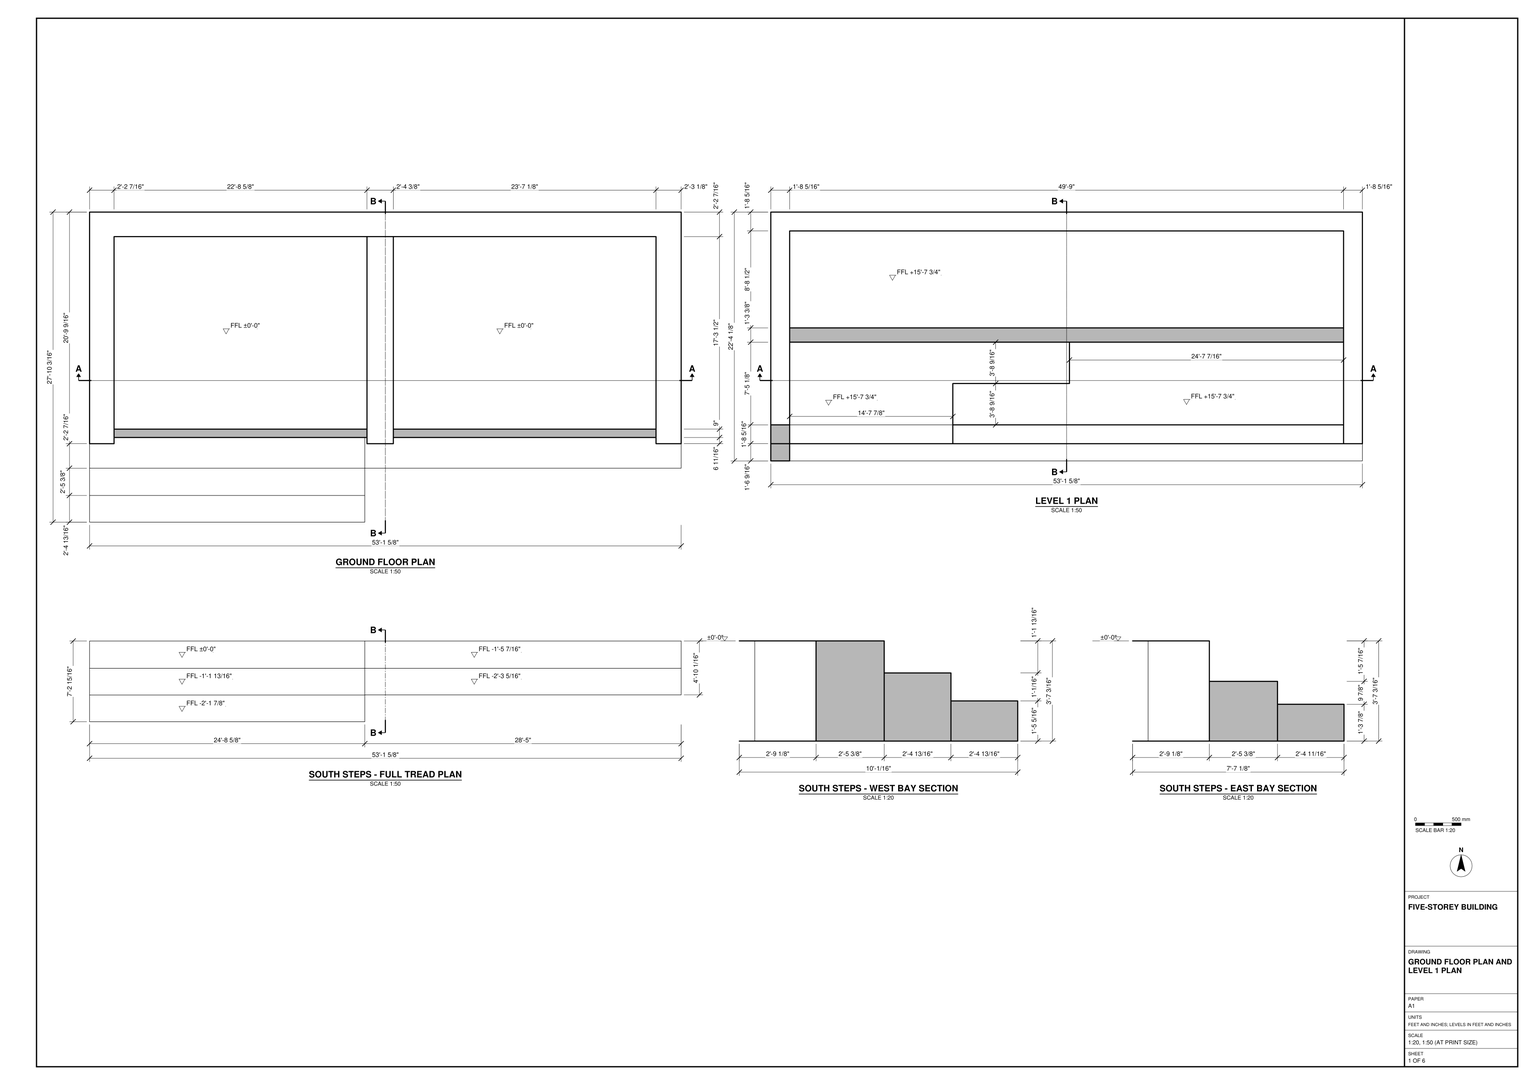
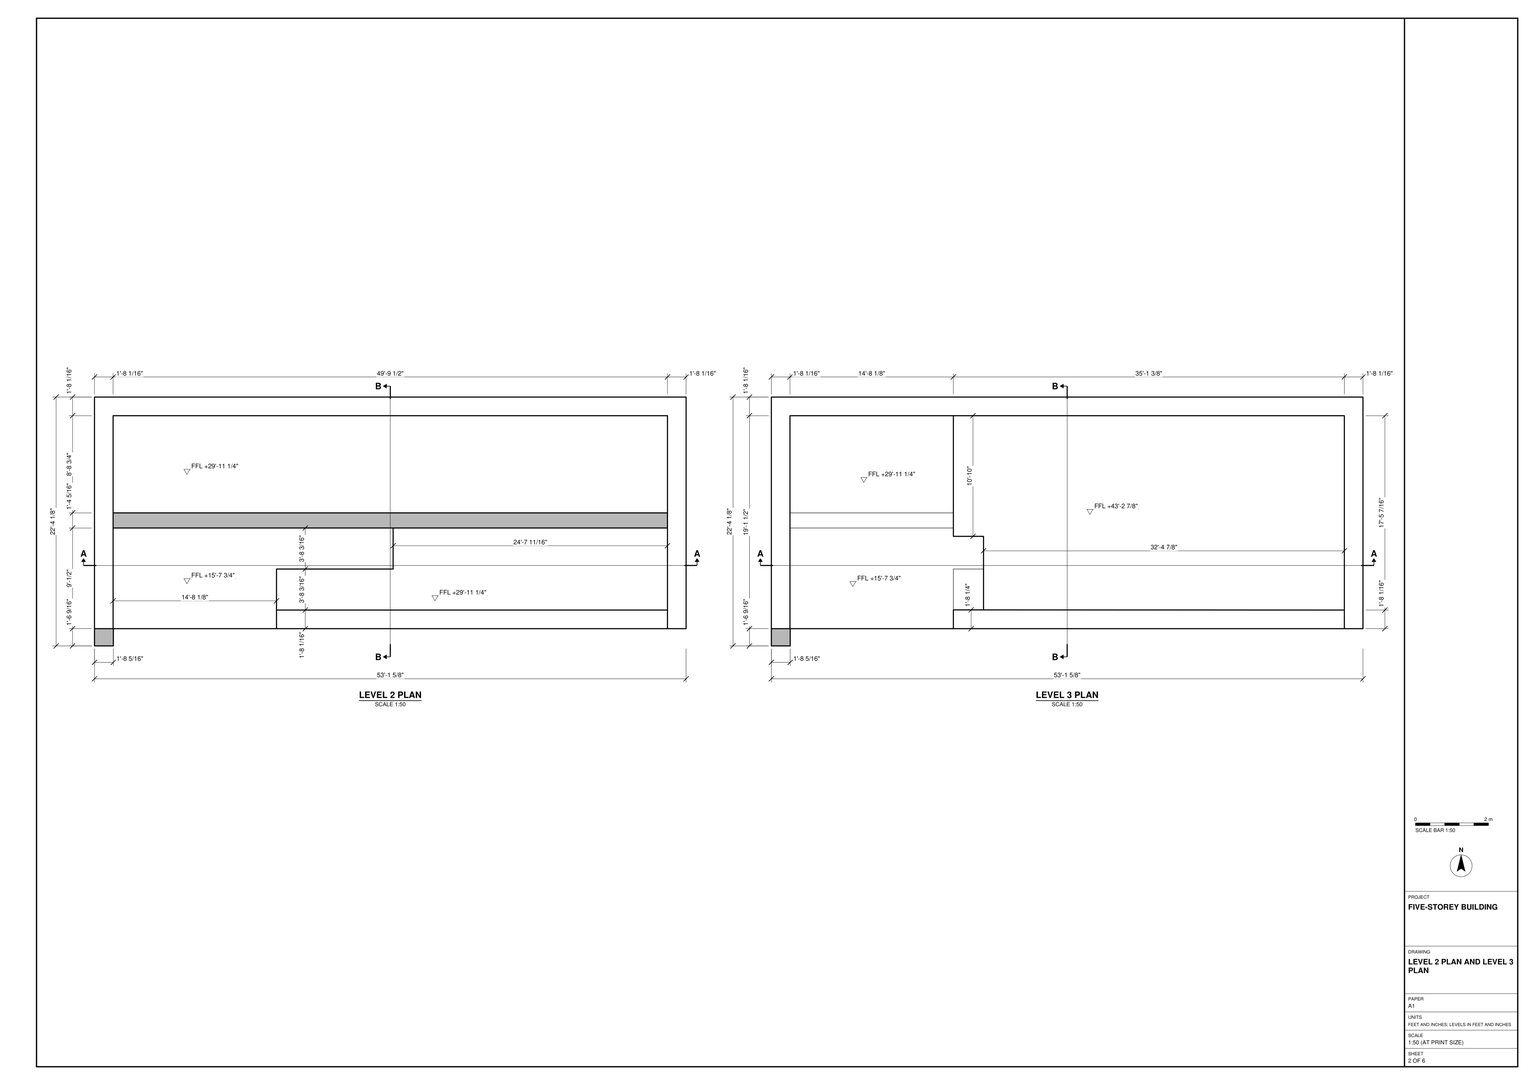
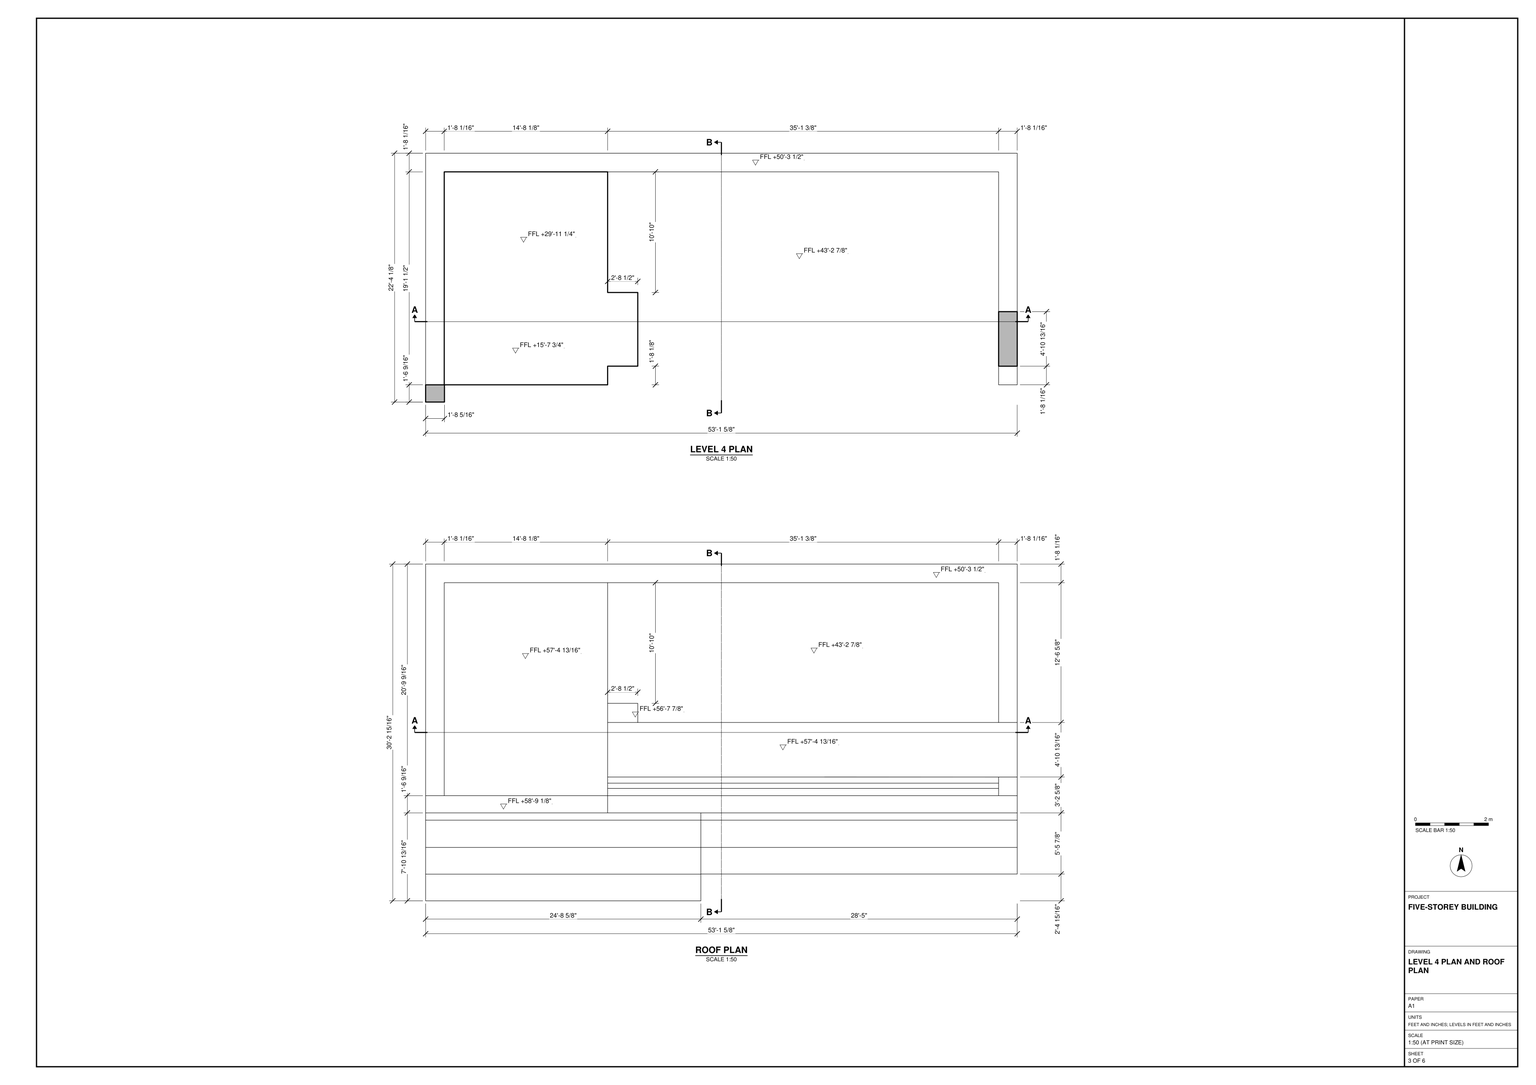
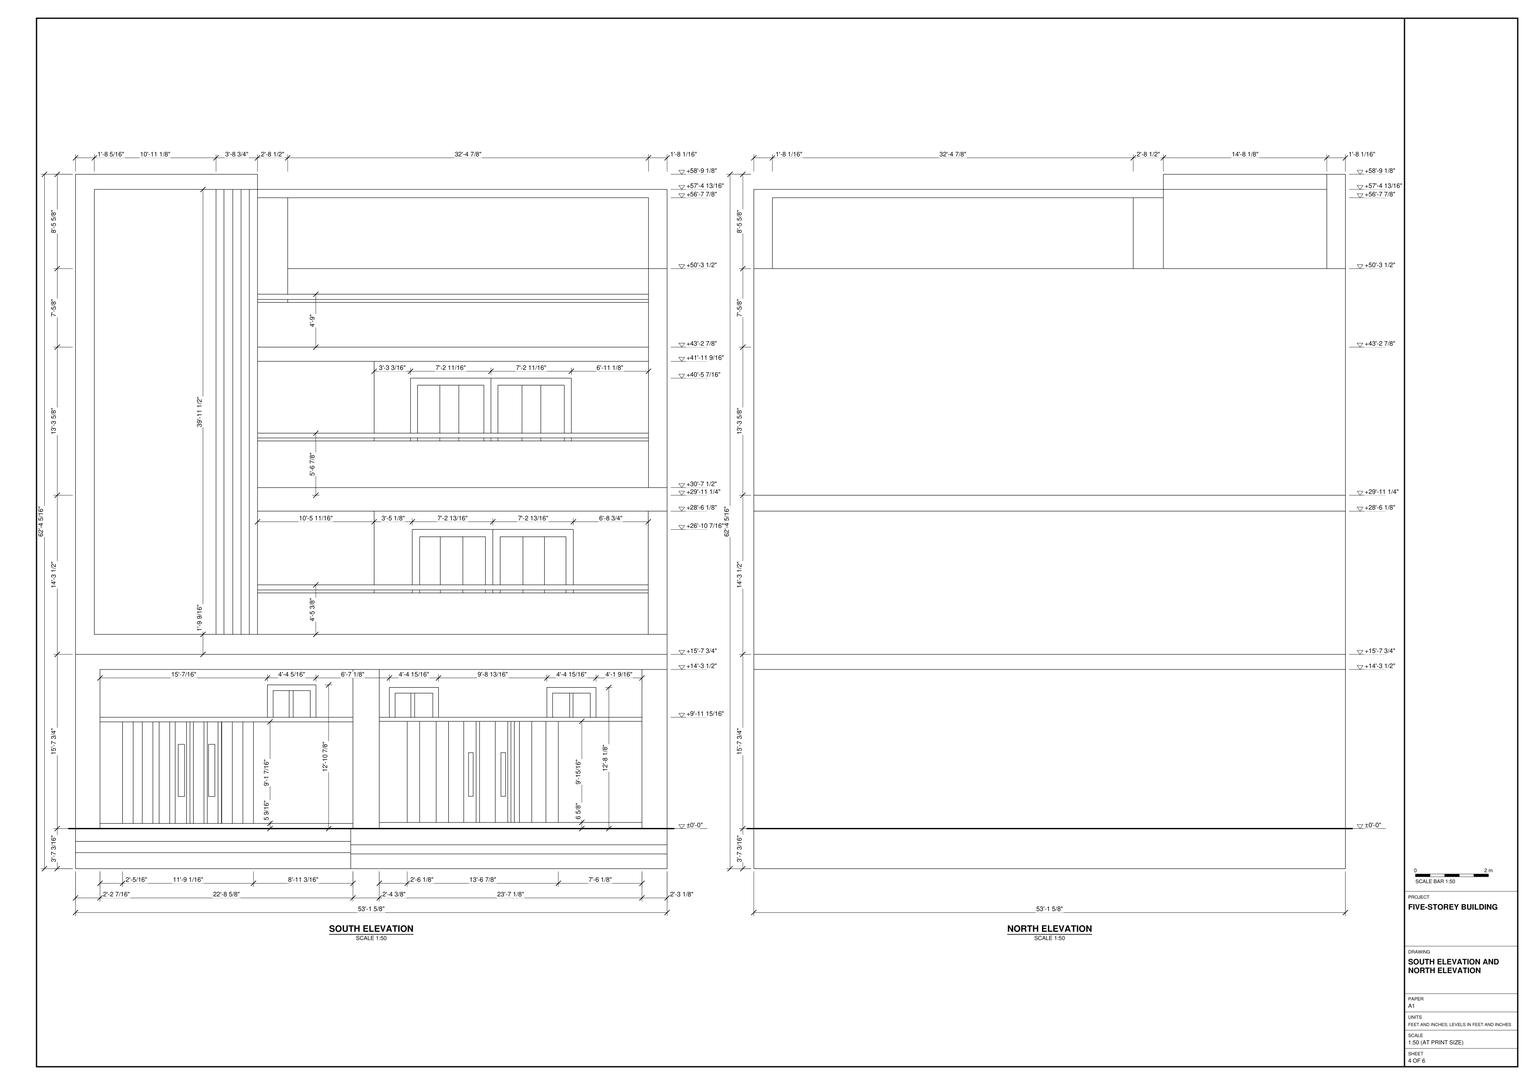
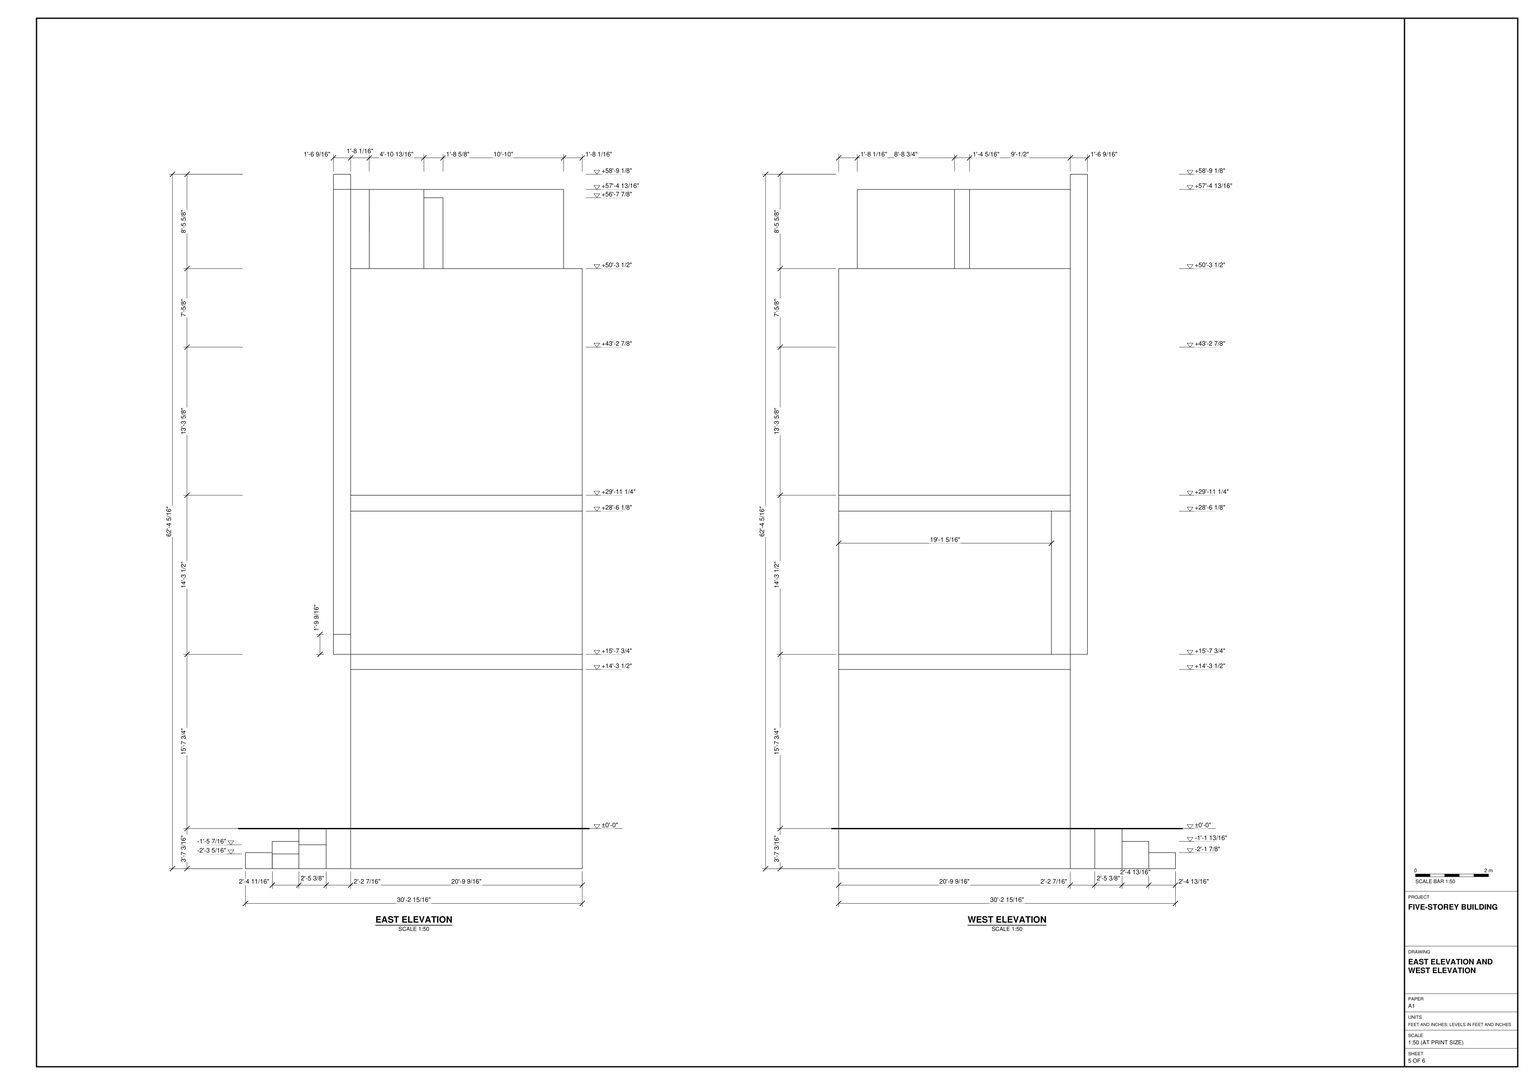
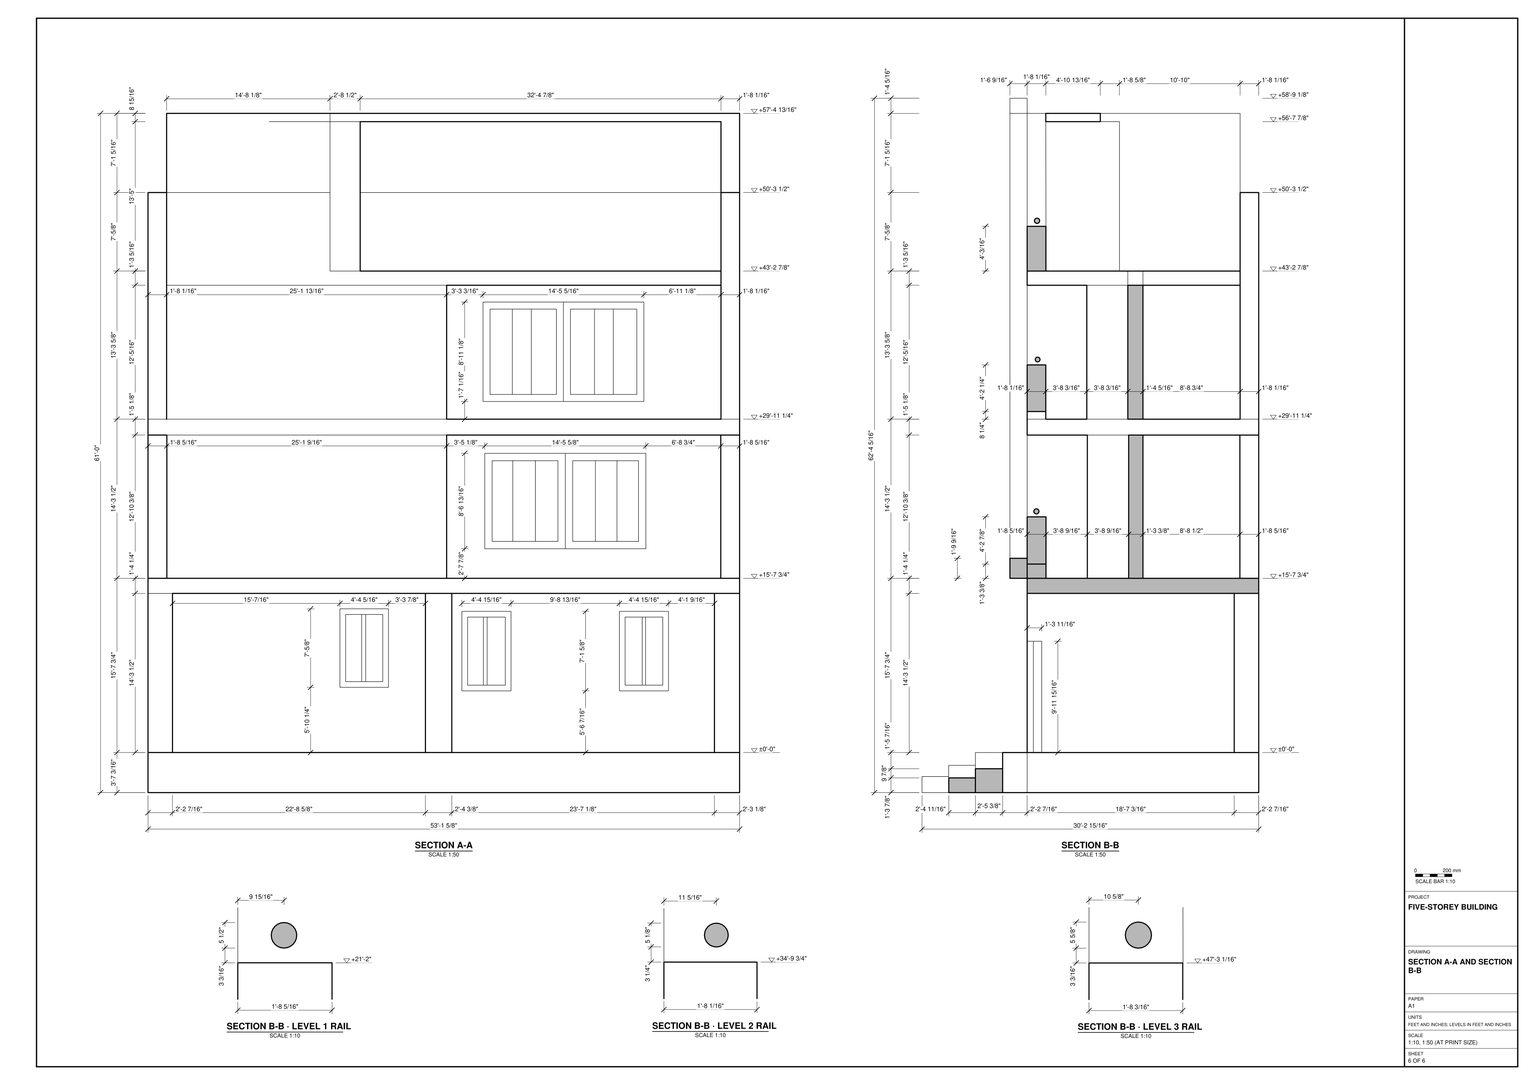
Build the five-storey building in SketchUp from task_files/diagram_01.pdf. Work in feet and inches. The overall extents, including the south steps, are 53'-1 5/8" east–west, 30'-2 15/16" north–south and 62'-4 5/16" vertically. Set the ground floor at ±0'-0" and Levels 1 through 4 at +15'-7 3/4", +29'-11 1/4", +43'-2 7/8" and +50'-3 1/2", respectively.

Start with the north wall, end walls and dividing wall that form the two ground-floor bays. Use the wall thicknesses drawn for each storey. At the south openings, use the tread plan for the footprint and the two bay sections for the tread heights; the west steps extend farther south than the east steps. Follow each upper plan separately for the slabs, walls and openings. Preserve the stepped slab edges and the lower floors visible through the upper levels. Form the roof over the west end and along the south side as drawn, rather than covering the entire footprint at one height.

Include built-in joinery and main furniture only where shown. Keep walls, slabs, steps, roof and each furniture or joinery piece in separate groups or components, and use components for repeated parts. Decor and loose items, where shown, may be any suitable library components. Save one SketchUp model as output_files/five_storey_building_with_stepped_south_access.skp.

# SketchUp Ruby script. Lengths in inches.
U = 1.inch
M = Sketchup.active_model
def pt(a) = Geom::Point3d.new(a.map { |v| v * U })
def face(e, loops, mat)
  f = e.add_face(loops[0].map { |a| pt(a) })
  loops[1..].each { |l| e.add_face(l.map { |a| pt(a) }).erase! }
  f.material = f.back_material = mat if mat
  f
end
# faces: each face lists its corners as indices into pts; further lists are holes
def faces(e, pts, list, mat = nil) = list.each { |f| face(e, (f[0].is_a?(Array) ? f : [f]).map { |l| l.map { |i| pts[i] } }, mat) }
# xy, xz, yz: faces in a plane at the given z, y or x. An outline is a flat list of corners, or four numbers for a rectangle; further outlines are holes
def ring(l) = l.size == 4 ? [[l[0], l[1]], [l[2], l[1]], [l[2], l[3]], [l[0], l[3]]] : l.each_slice(2).to_a
def flat(e, list, mat, &to3) = list.each { |f| face(e, (f[0].is_a?(Array) ? f : [f]).map { |l| ring(l).map { |u, v| to3.(u, v) } }, mat) }
def xy(e, z, list, mat = nil) = flat(e, list, mat) { |x, y| [x, y, z] }
def xz(e, y, list, mat = nil) = flat(e, list, mat) { |x, z| [x, y, z] }
def yz(e, x, list, mat = nil) = flat(e, list, mat) { |y, z| [x, y, z] }
def lines(e, pts, list) = list.each { |a, b| e.add_line(pt(pts[a]), pt(pts[b])) }
# prism: a flat outline (further loops are holes) pulled along v
def prism(e, loops, v, mat = nil)
  f = face(e, loops, mat); d = Geom::Vector3d.new(v.map { |x| x * U })
  f.pushpull(f.normal.samedirection?(d) ? d.length : -d.length)
end
def box(e, o, s, mat = nil) = prism(e, [[o, [o[0] + s[0], o[1], o[2]], [o[0] + s[0], o[1] + s[1], o[2]], [o[0], o[1] + s[1], o[2]]]], [0, 0, s[2]], mat)
def at(x, y, z, deg = 0) = Geom::Transformation.translation(pt([x, y, z])) * Geom::Transformation.rotation(ORIGIN, Z_AXIS, deg.degrees)
def axes(o, x, y, z) = Geom::Transformation.new([*x, 0, *y, 0, *z, 0, *pt(o).to_a, 1])
def part(name) = M.definitions.add(name)
# library, detail: a bought-in or finely detailed component or shape, given as its bounding box
def library(name, o, s) = part(name).tap { |d| box(d.entities, o, s) }
def detail(e, o, s) = box(e.add_group.entities, o, s)
def put(e, d, t, mat = nil) = e.add_instance(d, t).tap { |i| i.material = mat if mat }
def group(e, t, mat = nil) = e.add_group.tap { |g| g.transformation = t; g.material = mat if mat }.entities
root = M.entities
M.materials.add("[0035_Tan]").color = [191, 163, 127]
M.materials.add("[Blinds Cellular White]").color = [217, 211, 213]
M.materials.add("[Blinds Cloth Horizontal]").color = [192, 163, 85]
M.materials.add("[Formica Beige]").color = [211, 187, 149]
M.materials.add("[Formica Graystone]").color = [149, 146, 135]
M.materials.add("[Formica Laminate Light]").color = [213, 189, 164]
M.materials.add("[Formica Speckled Grey]").color = [94, 105, 111]
M.materials.add("[Granite Brown]").color = [126, 104, 91]
M.materials.add("[Quartz Light Brown]").color = [199, 184, 152]
M.materials.add("[Sketchy Scales]").color = [198, 170, 96]
M.materials.add("[Stone Brushed Khaki]").color = [226, 197, 133]
M.materials.add("[Terrazzo Tile Light]").color = [219, 217, 210]
M.materials.add("[Translucent Glass Safety]").color = [204, 235, 244]
M.materials["[Translucent Glass Safety]"].alpha = 0.5
M.materials.add("[Window Covering 02]").color = [199, 178, 115]
M.materials.add("[Wood Cherry Original]").color = [152, 86, 42]
M.materials.add("[Wood Veneer 01]").color = [81, 47, 25]
M.materials.add("[Wood Veneer 01]1").color = [120, 70, 37]
M.materials.add("[Wood Veneer 02]").color = [190, 128, 91]
xy(root,0,[[0,0,296.65,28.78],[0,28.78,296.65,57.57],[296.65,28.91,637.64,57.57],[0,57.57,296.65,86.95],[296.65,57.57,637.64,86.95],
  [0,86.95,637.64,362.96]])
xy(root,15.875,[[296.65,28.91,637.64,57.57]],"[Granite Brown]")
xy(root,17.3125,[[0,0,296.65,28.78]],"[Stone Brushed Khaki]")
xy(root,25.75,[[296.65,57.57,637.64,86.95]],"[Granite Brown]")
xy(root,29.375,[[0,28.78,296.65,57.57]],"[Stone Brushed Khaki]")
xy(root,43.1875,[[0,113.36,0,362.96,637.64,362.96,637.64,113.36,610.54,113.36,610.54,336.54,26.41,336.54,26.41,113.36],[299.03,113.36,327.42,336.54],[26.41,120.05,299.03,129.06],[327.42,120.05,610.54,129.06],[26.41,129.06,299.03,336.54],
  [327.42,129.06,610.54,336.54]])
xy(root,43.1875,[[296.65,86.95,637.64,86.95,637.64,113.36,610.54,113.36,610.54,120.05,327.42,120.05,327.42,113.36,299.03,113.36,299.03,120.05,296.65,120.05]],"[Granite Brown]")
xy(root,43.1875,[[0,57.57,296.65,86.95],[0,86.95,296.65,86.95,296.65,120.05,26.41,120.05,26.41,113.36,0,113.36]],"[Stone Brushed Khaki]")
xy(root,163.125,[[26.41,120.05,299.03,129.06],[327.42,120.05,610.54,129.06]],"[Wood Cherry Original]")
xy(root,214.6875,[[299.03,113.36,327.42,336.54],[610.54,113.36,637.64,362.96],[26.41,336.54,299.03,362.96],[299.03,336.54,327.42,362.96],[327.42,336.54,610.54,362.96]])
xy(root,214.6875,[[26.41,113.36,299.03,336.54],[327.42,113.36,610.54,336.54]],"[Formica Laminate Light]")
xy(root,230.9375,[[0,113.36,617.33,133.67],[617.33,113.36,617.33,342.65,20.31,342.65,20.31,133.67,0,133.67,0,362.96,637.64,362.96,637.64,113.36],[20.31,133.67,196.18,133.67,196.18,178.22,321.87,178.22,321.87,222.77,20.31,222.77],[196.18,133.67,617.33,133.67,617.33,222.77,321.87,222.77,321.87,178.22,196.18,178.22],[20.31,222.77,617.33,238.16],
  [20.31,238.16,617.33,342.65]])
xy(root,230.9375,[[0,94.8,637.64,113.36]],"[Wood Cherry Original]")
xy(root,246.3125,[[20.31,113.36,196.18,133.67],[196.18,113.36,617.33,133.67]])
xy(root,252.5,[[20.31,94.8,637.64,113.36]],"[Wood Cherry Original]")
xy(root,297.1875,[[196.18,113.36,617.33,133.67]])
xy(root,385.3125,[[0,113.36,20.31,133.67],[196.18,113.36,196.18,178.22,321.87,178.22,321.87,222.77,617.33,222.77,617.33,113.36],[617.33,113.36,637.64,222.77],[0,133.67,20.31,222.77],[0,222.77,20.31,238.16],
  [20.31,222.77,617.33,238.16],[617.33,222.77,637.64,238.16],[0,238.16,20.31,362.96],[20.31,238.16,617.33,342.65],[617.33,238.16,637.64,362.96],
  [20.31,342.65,617.33,362.96]])
xy(root,402.4375,[[196.18,133.43,617.57,133.43,617.57,221.86,321.87,221.86,321.87,177.65,196.18,177.65],[20.07,221.86,617.57,238.16],[20.07,238.16,617.57,342.89]])
xy(root,410.6875,[[196.18,113.36,617.57,133.43]])
xy(root,460.9375,[[196.18,113.36,617.57,133.43]])
xy(root,546.75,[[196.18,113.36,196.18,177.65,321.87,177.65,321.87,221.86,617.57,221.86,617.57,113.36],[20.07,221.86,617.57,238.16],[20.07,238.16,617.57,342.89]])
xy(root,562.0625,[[196.18,113.36,196.18,133.63,617.57,133.43,617.57,113.36],[617.57,133.43,617.57,342.89,196.18,342.89,196.18,212.87,228.68,212.87,228.68,133.63,196.18,133.63]])
xy(root,610.25,[[196.18,113.36,617.57,113.36,617.57,133.43,196.18,133.63]])
xy(root,646.6875,[[617.57,113.36,637.64,113.36,637.64,133.42,617.57,133.43],[637.64,133.42,617.57,133.43,617.57,192.24,637.64,192.24]])
xy(root,646.6875,[[0,113.36,20.07,113.36,20.07,342.89,617.57,342.89,617.57,192.24,637.64,192.24,637.64,362.96,0,362.96]],"[Formica Graystone]")
xy(root,723.08,[[228.68,133.43,617.57,192.24]])
xy(root,723.08,[[196.18,192.24,228.68,212.87]],"[Formica Laminate Light]")
xy(root,732,[[637.64,133.42,637.64,192.24,196.18,192.24,196.18,133.43]])
xy(root,732,[[20.07,113.36,196.18,342.89]],"[Formica Laminate Light]")
xy(root,732,[[20.31,94.8,196.18,113.36]],"[Wood Cherry Original]")
xy(root,748.3125,[[0,94.8,196.18,113.36]],"[Wood Cherry Original]")
xz(root,0,[[0,0,296.65,17.3125]],"[Stone Brushed Khaki]")
xz(root,28.78,[[0,0,296.65,17.3125]])
xz(root,28.78,[[0,17.3125,296.65,29.375]],"[Stone Brushed Khaki]")
xz(root,28.91,[[296.65,0,637.64,15.875]],"[Granite Brown]")
xz(root,57.57,[[0,0,296.65,29.375],[296.65,0,637.64,15.875]])
xz(root,57.57,[[296.65,15.875,637.64,25.75]],"[Granite Brown]")
xz(root,57.57,[[0,29.375,296.65,43.1875]],"[Stone Brushed Khaki]")
xz(root,86.95,[[0,0,296.65,43.1875],[296.65,0,637.64,25.75]])
xz(root,86.95,[[296.65,25.75,637.64,43.1875]],"[Granite Brown]")
xz(root,94.8,[[0,230.9375,637.64,230.9375,637.64,252.5,20.31,252.5,20.31,732,196.18,732,196.18,748.3125,0,748.3125]],"[Wood Cherry Original]")
xz(root,113.36,[[0,230.9375,0,385.3125,20.31,385.3125,20.31,246.3125,617.33,246.3125,617.33,230.9375],[617.33,230.9375,637.64,246.3125],[20.31,246.3125,196.18,252.5],[196.18,246.3125,617.33,252.5],[617.33,246.3125,637.64,252.5],
  [617.33,252.5,637.64,385.3125],[0,385.3125,20.31,402.4375],[0,402.4375,20.07,646.6875],[20.07,402.4375,20.31,732],[617.57,410.6875,637.64,646.6875],
  [196.18,546.75,617.57,562.0625]])
xz(root,113.36,[[0,43.1875,26.41,43.1875,26.41,214.6875,637.64,214.6875,637.64,230.9375,0,230.9375],[299.03,43.1875,327.42,214.6875],[610.54,43.1875,637.64,214.6875]],"[0035_Tan]")
xz(root,113.36,[[151.46,252.5,160.02,732],[160.02,252.5,169.52,732],[169.52,252.5,178.46,732],[178.46,252.5,187.32,732],[187.32,252.5,196.18,732]],"[Quartz Light Brown]")
xz(root,113.36,[[20.31,252.5,151.46,732]],"[Sketchy Scales]")
xz(root,113.36,[[196.18,252.5,617.33,297.1875],[196.18,410.6875,617.57,460.9375],[196.18,562.0625,617.57,610.25]],"[Translucent Glass Safety]")
xz(root,113.36,[[196.18,385.3125,637.64,410.6875],[0,646.6875,20.07,748.3125],[20.07,732,196.18,748.3125]],"[Wood Cherry Original]")
xz(root,120.05,[[157.31,48.74,157.66,158.18]])
xz(root,120.05,[[110.71,77.78,117.52,133.97],[143.4,77.78,150.21,133.97],[423.6,77.97,428.6,125.04],[458.54,77.97,463.54,125.04]],"[Formica Graystone]")
xz(root,120.05,[[26.41,43.1875,299.03,48.74],[327.42,43.1875,610.54,49.82],[26.41,158.18,299.03,163.125],[327.42,158.77,610.54,163.125]],"[Wood Cherry Original]")
xz(root,120.05,[[26.41,48.74,50.76,158.18],[62.16,48.74,72.01,158.18],[83.41,48.74,90.15,158.18],[101.56,48.74,107.48,158.18],[119.7,48.74,123.37,158.18],
  [123.37,48.74,127.1,158.18],[138.5,48.74,142.1,158.18],[153.63,48.74,157.31,158.18],[169.07,48.74,180.41,158.18],[191.82,48.74,299.03,158.18],
  [327.42,49.82,357.55,158.77],[370.91,49.82,388.74,158.77],[402.1,49.82,418.46,158.77],[431.82,49.82,435.5,158.77],[435.5,49.82,452.49,158.77],
  [465.85,49.82,469.32,158.77],[469.32,49.82,473,158.77],[473,49.82,478.43,158.77],[491.79,49.82,507.05,158.77],[520.41,49.82,610.54,158.77]],"[Wood Veneer 01]1")
xz(root,120.05,[[50.76,48.74,62.16,158.18],[72.01,48.74,83.41,158.18],[90.15,48.74,101.56,158.18],[[107.48,48.74,119.7,158.18],[110.71,77.78,117.52,133.97]],[127.1,48.74,138.5,158.18],
  [[142.1,48.74,153.63,158.18],[143.4,77.78,150.21,133.97]],[157.66,48.74,169.07,158.18],[180.41,48.74,191.82,158.18],[357.55,49.82,370.91,158.77],[388.74,49.82,402.1,158.77],
  [[418.46,49.82,431.82,158.77],[423.6,77.97,428.6,125.04]],[[452.49,49.82,465.85,158.77],[458.54,77.97,463.54,125.04]],[478.43,49.82,491.79,158.77],[507.05,49.82,520.41,158.77]],"[Wood Veneer 02]")
xz(root,129.06,[[26.41,43.1875,299.03,163.125],[327.42,43.1875,610.54,163.125]])
xz(root,133.43,[[196.18,402.4375,617.57,410.6875]])
xz(root,133.43,[[196.18,410.6875,617.57,460.9375]],"[Translucent Glass Safety]")
xz(root,133.63,[[196.18,562.0625,228.68,610.25]])
xz(root,133.67,[[0,230.9375,20.31,385.3125],[20.31,230.9375,196.18,246.3125],[196.18,230.9375,617.33,246.3125]])
xz(root,133.67,[[196.18,246.3125,617.33,297.1875]],"[Translucent Glass Safety]")
xz(root,177.65,[[196.18,402.4375,321.87,546.75]],"[Formica Laminate Light]")
xz(root,178.22,[[196.18,230.9375,321.87,385.3125]],"[Formica Laminate Light]")
xz(root,192.24,[[617.57,646.6875,617.57,723.08,196.18,723.08,196.18,732,637.64,732,637.64,646.6875]])
xz(root,212.87,[[196.18,562.0625,228.68,723.08]],"[Formica Laminate Light]")
xz(root,221.86,[[20.07,402.4375,321.87,546.75]])
xz(root,221.86,[[392.6875,429.08,413.15,521.07],[481.24,429.08,501.51,521.07]],"[Blinds Cellular White]")
xz(root,221.86,[[[321.87,402.4375,617.57,546.75],[361.09,421.51,534.42,528.64]]],"[Formica Laminate Light]")
xz(root,221.86,[[368.65,429.08,392.6875,521.07],[413.15,429.08,440.1875,521.07],[455.32,429.08,481.24,521.07],[501.51,429.08,526.85,521.07]],"[Window Covering 02]")
xz(root,221.86,[[[361.09,421.51,447.75,528.64],[368.65,429.08,440.1875,521.07]],[[447.75,421.51,534.42,528.64],[455.32,429.08,526.85,521.07]]],"[Wood Veneer 01]")
xz(root,222.77,[[20.31,230.9375,321.87,385.3125]])
xz(root,222.77,[[393.17,270.74,417.51,357.68],[482.24,270.74,505.46,357.68]],"[Blinds Cellular White]")
xz(root,222.77,[[370.91,270.74,393.17,357.68],[417.51,270.74,441.85,357.68],[457.73,270.74,482.24,357.68],[505.46,270.74,528.67,357.68]],"[Blinds Cloth Horizontal]")
xz(root,222.77,[[[321.87,230.9375,617.33,385.3125],[362.98,262.8,536.6,365.61]]],"[Formica Laminate Light]")
xz(root,222.77,[[[362.98,262.8,449.79,365.61],[370.91,270.74,441.85,357.68]],[[449.79,262.8,536.6,365.61],[457.73,270.74,528.67,357.68]]],"[Wood Veneer 01]")
xz(root,238.16,[[20.31,230.9375,617.33,385.3125],[20.07,402.4375,617.57,546.75]])
xz(root,336.54,[[299.03,43.1875,327.42,214.6875]])
xz(root,336.54,[[[26.41,43.1875,299.03,214.6875],[206.86,113.44,259.18,198.09]],[[327.42,43.1875,610.54,214.6875],[338.3125,109.64,391.25,195.3],[508.0625,109.64,561,195.3]]],"[Formica Speckled Grey]")
xz(root,336.54,[[[338.3125,109.64,391.25,195.3],[344.46,115.79,385.1,189.15]],[[508.0625,109.64,561,195.3],[514.21,115.79,554.85,189.15]],[[206.86,113.44,259.18,198.09],[213.01,119.59,253.03,191.9375]],[361.48,115.79,365.53,189.15],[532.64,115.79,536.27,189.15],
  [230.29,119.59,234.625,191.9375]],"[Wood Veneer 01]1")
xz(root,336.54,[[344.46,115.79,361.48,189.15],[365.53,115.79,385.1,189.15],[514.21,115.79,532.64,189.15],[536.27,115.79,554.85,189.15],[213.01,119.59,230.29,191.9375],
  [234.625,119.59,253.03,191.9375]],"[Wood Veneer 02]")
xz(root,342.65,[[20.31,230.9375,617.33,385.3125]])
xz(root,342.89,[[20.07,402.4375,617.57,546.75],[20.07,546.75,617.57,546.75,617.57,562.0625,196.18,562.0625,196.18,646.6875,20.07,646.6875]])
xz(root,342.89,[[20.07,646.6875,196.18,732]],"[Formica Graystone]")
xz(root,342.89,[[196.18,562.0625,617.57,646.6875]],"[Quartz Light Brown]")
xz(root,362.96,[[0,0,637.64,43.1875],[0,43.1875,637.64,214.6875],[0,214.6875,637.64,230.9375],[0,230.9375,637.64,385.3125],[0,385.3125,637.64,402.4375],
  [0,402.4375,637.64,646.6875]],"[Formica Beige]")
yz(root,0,[[113.36,0,362.96,43.1875],[113.36,43.1875,362.96,214.6875],[113.36,214.6875,362.96,230.9375],[113.36,230.9375,133.67,385.3125],[133.67,230.9375,362.96,385.3125],
  [113.36,385.3125,362.96,402.4375],[113.36,402.4375,362.96,646.6875]],"[Formica Beige]")
yz(root,0,[[0,0,28.78,17.3125],[28.78,0,57.57,29.375],[57.57,0,86.95,43.1875],[86.95,0,113.36,43.1875]],"[Stone Brushed Khaki]")
yz(root,0,[[94.8,230.9375,113.36,748.3125]],"[Wood Cherry Original]")
yz(root,20.07,[[113.36,402.4375,221.86,546.75],[221.86,402.4375,238.16,546.75],[238.16,402.4375,342.89,546.75],[113.36,546.75,221.86,646.6875],[221.86,546.75,238.16,646.6875],
  [238.16,546.75,342.89,646.6875]])
yz(root,20.07,[[113.36,646.6875,221.86,732],[221.86,646.6875,238.16,732],[238.16,646.6875,342.89,732]],"[Formica Graystone]")
yz(root,20.31,[[133.67,230.9375,222.77,385.3125],[222.77,230.9375,238.16,385.3125],[238.16,230.9375,342.65,385.3125],[113.36,246.3125,133.67,385.3125]])
yz(root,20.31,[[94.8,252.5,113.36,732]],"[Wood Cherry Original]")
yz(root,26.41,[[120.05,43.1875,129.06,163.125]])
yz(root,26.41,[[113.36,43.1875,120.05,163.125],[129.06,43.1875,336.54,43.1875,336.54,214.6875,113.36,214.6875,113.36,163.125,129.06,163.125]],"[0035_Tan]")
yz(root,196.18,[[113.36,246.3125,133.67,297.1875],[123.32,300.36,122.61,300.46,121.94,300.73,121.375,301.17,120.9375,301.74,120.66,302.4,120.57,303.11,120.66,303.83,120.9375,304.49,121.375,305.06,121.94,305.49,122.61,305.77,123.32,305.86,124.03,305.77,124.69,305.49,125.26,305.06,125.7,304.49,125.98,303.83,126.07,303.11,125.98,302.4,125.7,301.74,125.26,301.17,124.69,300.73,124.03,300.46],[113.36,410.6875,133.43,460.9375],[113.36,562.0625,133.63,610.25]])
yz(root,196.18,[[[133.67,230.9375,178.22,230.9375,178.22,385.3125,113.36,385.3125,113.36,297.1875,133.67,297.1875],[123.32,300.36,122.61,300.46,121.94,300.73,121.375,301.17,120.9375,301.74,120.66,302.4,120.57,303.11,120.66,303.83,120.9375,304.49,121.375,305.06,121.94,305.49,122.61,305.77,123.32,305.86,124.03,305.77,124.69,305.49,125.26,305.06,125.7,304.49,125.98,303.83,126.07,303.11,125.98,302.4,125.7,301.74,125.26,301.17,124.69,300.73,124.03,300.46]],[[133.43,402.4375,177.65,402.4375,177.65,546.75,113.36,546.75,113.36,460.9375,133.43,460.9375],[124.66,464.2,124,464.29,123.38,464.55,122.85,464.95,122.44,465.48,122.1875,466.1,122.1,466.77,122.1875,467.43,122.44,468.05,122.85,468.58,123.38,468.98,124,469.24,124.66,469.33,125.33,469.24,125.94,468.98,126.47,468.58,126.88,468.05,127.14,467.43,127.22,466.77,127.14,466.1,126.88,465.48,126.47,464.95,125.94,464.55,125.33,464.29]],[212.87,562.0625,342.89,562.0625,342.89,732,192.24,732,192.24,723.08,212.87,723.08],[[113.36,610.25,133.63,610.25,133.43,723.08,133.43,732,113.36,732],[124.01,613.45,123.28,613.55,122.61,613.83,122.02,614.28,121.58,614.86,121.3,615.54,121.2,616.27,121.3,616.99,121.58,617.67,122.02,618.25,122.61,618.7,123.28,618.98,124.01,619.08,124.74,618.98,125.42,618.7,126,618.25,126.45,617.67,126.73,616.99,126.82,616.27,126.73,615.54,126.45,614.86,126,614.28,125.42,613.83,124.74,613.55]]],"[Formica Laminate Light]")
yz(root,196.18,[[94.8,732,113.36,748.3125]],"[Wood Cherry Original]")
yz(root,228.68,[[133.63,562.0625,212.87,562.0625,212.87,723.08,133.43,723.08,133.63,610.25]],"[Formica Laminate Light]")
yz(root,296.65,[[0,0,28.78,17.3125],[28.78,0,28.91,0,28.91,15.875,57.57,15.875,57.57,29.375,28.78,29.375],[28.91,0,57.57,15.875],[57.57,0,86.95,25.75],[57.57,25.75,86.95,43.1875]])
yz(root,299.03,[[120.05,43.1875,129.06,163.125]])
yz(root,299.03,[[113.36,43.1875,120.05,163.125],[129.06,43.1875,129.06,163.125,113.36,163.125,113.36,214.6875,336.54,214.6875,336.54,43.1875]],"[0035_Tan]")
yz(root,321.87,[[178.22,230.9375,222.77,385.3125],[177.65,402.4375,221.86,546.75]],"[Formica Laminate Light]")
yz(root,327.42,[[120.05,43.1875,129.06,163.125]])
yz(root,327.42,[[113.36,43.1875,120.05,43.1875,120.05,163.125,129.06,163.125,129.06,43.1875,336.54,43.1875,336.54,214.6875,113.36,214.6875]],"[0035_Tan]")
yz(root,610.54,[[120.05,43.1875,129.06,163.125]])
yz(root,610.54,[[113.36,43.1875,120.05,163.125],[129.06,43.1875,129.06,163.125,113.36,163.125,113.36,214.6875,336.54,214.6875,336.54,43.1875]],"[0035_Tan]")
yz(root,617.33,[[113.36,230.9375,133.67,246.3125],[[133.67,230.9375,133.67,297.1875,113.36,297.1875,113.36,385.3125,222.77,385.3125,222.77,230.9375],[123.32,300.36,124.03,300.46,124.69,300.73,125.26,301.17,125.7,301.74,125.98,302.4,126.07,303.11,125.98,303.83,125.7,304.49,125.26,305.06,124.69,305.49,124.03,305.77,123.32,305.86,122.61,305.77,121.94,305.49,121.375,305.06,120.9375,304.49,120.66,303.83,120.57,303.11,120.66,302.4,120.9375,301.74,121.375,301.17,121.94,300.73,122.61,300.46]],[222.77,230.9375,238.16,385.3125],[238.16,230.9375,342.65,385.3125],[113.36,246.3125,133.67,297.1875]])
yz(root,617.57,[[133.43,402.4375,221.86,546.75],[221.86,402.4375,238.16,546.75],[238.16,402.4375,342.89,546.75],[113.36,410.6875,133.43,460.9375],[[113.36,460.9375,133.43,546.75],[124.66,464.2,125.33,464.29,125.94,464.55,126.47,464.95,126.88,465.48,127.14,466.1,127.22,466.77,127.14,467.43,126.88,468.05,126.47,468.58,125.94,468.98,125.33,469.24,124.66,469.33,124,469.24,123.38,468.98,122.85,468.58,122.44,468.05,122.1875,467.43,122.1,466.77,122.1875,466.1,122.44,465.48,122.85,464.95,123.38,464.55,124,464.29]],
  [124.66,464.2,125.33,464.29,125.94,464.55,126.47,464.95,126.88,465.48,127.14,466.1,127.22,466.77,127.14,467.43,126.88,468.05,126.47,468.58,125.94,468.98,125.33,469.24,124.66,469.33,124,469.24,123.38,468.98,122.85,468.58,122.44,468.05,122.1875,467.43,122.1,466.77,122.1875,466.1,122.44,465.48,122.85,464.95,123.38,464.55,124,464.29],[113.36,546.75,133.43,562.0625],[133.43,546.75,221.86,562.0625],[221.86,546.75,238.16,562.0625],[238.16,546.75,342.89,562.0625],
  [113.36,562.0625,133.43,610.25],[124.01,613.45,124.74,613.55,125.42,613.83,126,614.28,126.45,614.86,126.73,615.54,126.82,616.27,126.73,616.99,126.45,617.67,126,618.25,125.42,618.7,124.74,618.98,124.01,619.08,123.28,618.98,122.61,618.7,122.02,618.25,121.58,617.67,121.3,616.99,121.2,616.27,121.3,615.54,121.58,614.86,122.02,614.28,122.61,613.83,123.28,613.55],[133.43,646.6875,192.24,723.08]])
yz(root,617.57,[[133.43,562.0625,342.89,646.6875],[[113.36,610.25,133.43,646.6875],[124.01,613.45,124.74,613.55,125.42,613.83,126,614.28,126.45,614.86,126.73,615.54,126.82,616.27,126.73,616.99,126.45,617.67,126,618.25,125.42,618.7,124.74,618.98,124.01,619.08,123.28,618.98,122.61,618.7,122.02,618.25,121.58,617.67,121.3,616.99,121.2,616.27,121.3,615.54,121.58,614.86,122.02,614.28,122.61,613.83,123.28,613.55]]],"[Quartz Light Brown]")
yz(root,637.64,[[133.42,646.6875,192.24,732]])
yz(root,637.64,[[113.36,0,362.96,43.1875],[113.36,43.1875,362.96,214.6875],[113.36,214.6875,362.96,230.9375],[113.36,230.9375,362.96,385.3125],[113.36,385.3125,362.96,402.4375],
  [113.36,402.4375,362.96,646.6875]],"[Formica Beige]")
yz(root,637.64,[[28.91,0,57.57,15.875],[57.57,0,86.95,25.75],[86.95,0,113.36,43.1875]],"[Granite Brown]")
yz(root,637.64,[[94.8,230.9375,113.36,252.5]],"[Wood Cherry Original]")
p = [[196.18,122.61,300.46],[196.18,123.32,300.36],[617.33,123.32,300.36],[617.33,122.61,300.46],[196.18,124.03,300.46],[617.33,124.03,300.46],
  [196.18,121.94,300.73],[617.33,121.94,300.73],[196.18,124.69,300.73],[617.33,124.69,300.73],[196.18,121.375,301.17],[617.33,121.375,301.17],
  [196.18,125.26,301.17],[617.33,125.26,301.17],[196.18,120.9375,301.74],[617.33,120.9375,301.74],[196.18,125.7,301.74],[617.33,125.7,301.74],
  [196.18,120.66,302.4],[617.33,120.66,302.4],[196.18,125.98,302.4],[617.33,125.98,302.4],[196.18,120.57,303.11],[617.33,120.57,303.11],
  [196.18,126.07,303.11],[617.33,126.07,303.11],[196.18,120.66,303.83],[617.33,120.66,303.83],[196.18,125.98,303.83],[617.33,125.98,303.83],
  [196.18,120.9375,304.49],[617.33,120.9375,304.49],[196.18,125.7,304.49],[617.33,125.7,304.49],[196.18,121.375,305.06],[617.33,121.375,305.06],
  [196.18,125.26,305.06],[617.33,125.26,305.06],[196.18,121.94,305.49],[617.33,121.94,305.49],[196.18,124.69,305.49],[617.33,124.69,305.49],
  [196.18,122.61,305.77],[617.33,122.61,305.77],[196.18,124.03,305.77],[617.33,124.03,305.77],[196.18,123.32,305.86],[617.33,123.32,305.86],
  [617.57,124.66,464.2],[617.57,124,464.29],[196.18,124,464.29],[196.18,124.66,464.2],[617.57,125.33,464.29],[196.18,125.33,464.29],
  [617.57,123.38,464.55],[196.18,123.38,464.55],[617.57,125.94,464.55],[196.18,125.94,464.55],[617.57,122.85,464.95],[196.18,122.85,464.95],
  [617.57,126.47,464.95],[196.18,126.47,464.95],[617.57,122.44,465.48],[196.18,122.44,465.48],[617.57,126.88,465.48],[196.18,126.88,465.48],
  [617.57,122.1875,466.1],[196.18,122.1875,466.1],[617.57,127.14,466.1],[196.18,127.14,466.1],[617.57,122.1,466.77],[196.18,122.1,466.77],
  [617.57,127.22,466.77],[196.18,127.22,466.77],[617.57,122.1875,467.43],[196.18,122.1875,467.43],[617.57,127.14,467.43],[196.18,127.14,467.43],
  [617.57,122.44,468.05],[196.18,122.44,468.05],[617.57,126.88,468.05],[196.18,126.88,468.05],[617.57,122.85,468.58],[196.18,122.85,468.58],
  [617.57,126.47,468.58],[196.18,126.47,468.58],[617.57,123.38,468.98],[196.18,123.38,468.98],[617.57,125.94,468.98],[196.18,125.94,468.98],
  [617.57,124,469.24],[196.18,124,469.24],[617.57,125.33,469.24],[196.18,125.33,469.24],[617.57,124.66,469.33],[196.18,124.66,469.33],
  [617.57,133.43,562.0625],[196.18,133.63,562.0625],[196.18,133.63,610.25],[617.57,133.43,610.25],[196.18,133.43,723.08],[228.68,133.63,610.25],
  [228.68,133.43,723.08],[617.57,123.28,613.55],[617.57,122.61,613.83],[196.18,122.61,613.83],[196.18,123.28,613.55],[617.57,124.01,613.45],
  [196.18,124.01,613.45],[617.57,124.74,613.55],[196.18,124.74,613.55],[617.57,125.42,613.83],[196.18,125.42,613.83],[617.57,122.02,614.28],
  [196.18,122.02,614.28],[617.57,126,614.28],[196.18,126,614.28],[617.57,121.58,614.86],[196.18,121.58,614.86],[617.57,126.45,614.86],
  [196.18,126.45,614.86],[617.57,121.3,615.54],[196.18,121.3,615.54],[617.57,126.73,615.54],[196.18,126.73,615.54],[617.57,121.2,616.27],
  [196.18,121.2,616.27],[617.57,126.82,616.27],[196.18,126.82,616.27],[617.57,121.3,616.99],[196.18,121.3,616.99],[617.57,126.73,616.99],
  [196.18,126.73,616.99],[617.57,121.58,617.67],[196.18,121.58,617.67],[617.57,126.45,617.67],[196.18,126.45,617.67],[617.57,122.02,618.25],
  [196.18,122.02,618.25],[617.57,126,618.25],[196.18,126,618.25],[617.57,122.61,618.7],[196.18,122.61,618.7],[617.57,125.42,618.7],
  [196.18,125.42,618.7],[617.57,123.28,618.98],[196.18,123.28,618.98],[617.57,124.74,618.98],[196.18,124.74,618.98],[617.57,124.01,619.08],
  [196.18,124.01,619.08],[637.64,133.42,646.6875],[637.64,133.42,732],[617.57,133.43,646.6875],[617.57,133.43,723.08],[196.18,133.43,732],
  [617.57,133.43,402.4375],[617.57,113.36,402.4375],[196.18,192.24,723.08],[130.5,192.24,723.08]]
faces(root,p,[[0,1,2,3],[1,4,5,2],[6,0,3,7],[4,8,9,5],[10,6,7,11],[8,12,13,9],[14,10,11,15],[12,16,17,13],
  [18,14,15,19],[16,20,21,17],[22,18,19,23],[20,24,25,21],[26,22,23,27],[24,28,29,25],[30,26,27,31],[28,32,33,29],
  [34,30,31,35],[32,36,37,33],[38,34,35,39],[36,40,41,37],[42,38,39,43],[40,44,45,41],[46,42,43,47],[44,46,47,45],
  [48,49,50,51],[52,48,51,53],[49,54,55,50],[56,52,53,57],[54,58,59,55],[60,56,57,61],[58,62,63,59],[64,60,61,65],
  [62,66,67,63],[68,64,65,69],[66,70,71,67],[72,68,69,73],[70,74,75,71],[76,72,73,77],[74,78,79,75],[80,76,77,81],
  [78,82,83,79],[84,80,81,85],[82,86,87,83],[88,84,85,89],[86,90,91,87],[92,88,89,93],[90,94,95,91],[94,92,93,95],
  [103,104,105,106],[107,103,106,108],[109,107,108,110],[111,109,110,112],[104,113,114,105],[115,111,112,116],[113,117,118,114],[119,115,116,120],
  [117,121,122,118],[123,119,120,124],[121,125,126,122],[127,123,124,128],[125,129,130,126],[131,127,128,132],[129,133,134,130],[135,131,132,136],
  [133,137,138,134],[139,135,136,140],[137,141,142,138],[143,139,140,144],[141,145,146,142],[147,143,144,148],[145,149,150,146],[149,147,148,150]],"[Terrazzo Tile Light]")
faces(root,p,[[96,97,98,99]],"[Translucent Glass Safety]")
faces(root,p,[[100,98,101,102]],"[Formica Laminate Light]")
faces(root,p,[[151,152,153],[154,153,152],[102,154,152,100],[155,100,152]])
lines(root,p,[[156,157],[158,159]])
